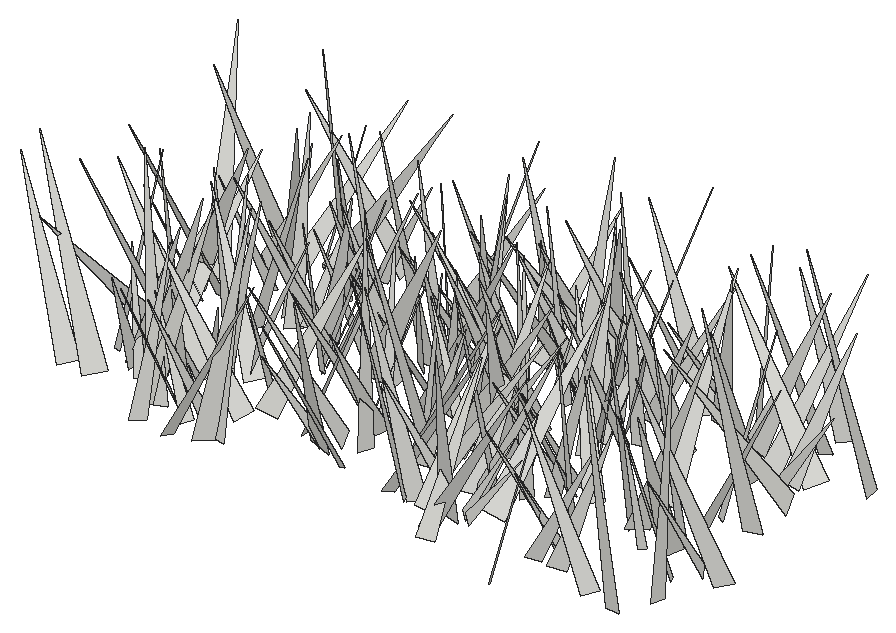
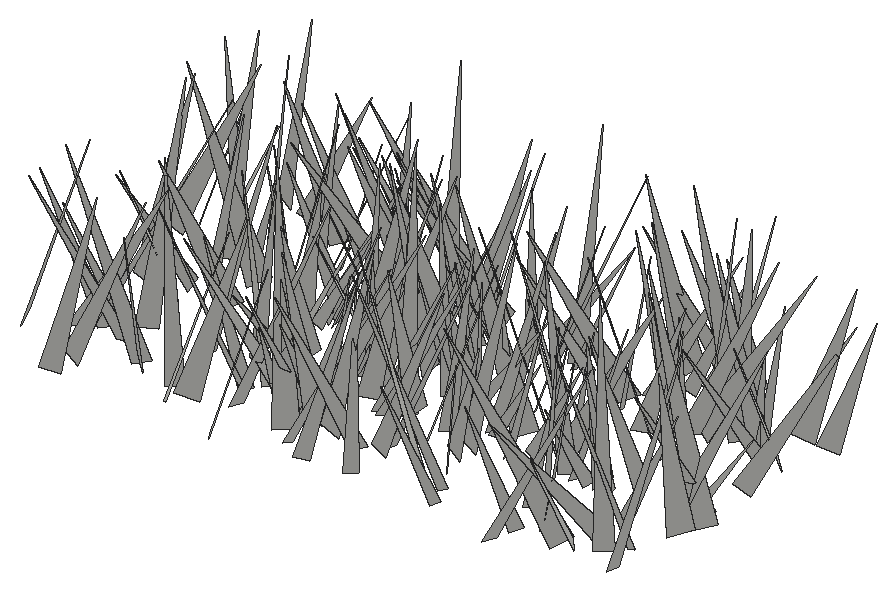
# SketchUp Ruby script. Lengths in inches.
U = 1.inch
M = Sketchup.active_model
def pt(a) = Geom::Point3d.new(a.map { |v| v * U })
def face(e, loops, mat)
  f = e.add_face(loops[0].map { |a| pt(a) })
  loops[1..].each { |l| e.add_face(l.map { |a| pt(a) }).erase! }
  f.material = f.back_material = mat if mat
  f
end
# faces: each face lists its corners as indices into pts; further lists are holes
def faces(e, pts, list, mat = nil) = list.each { |f| face(e, (f[0].is_a?(Array) ? f : [f]).map { |l| l.map { |i| pts[i] } }, mat) }
# xy, xz, yz: faces in a plane at the given z, y or x. An outline is a flat list of corners, or four numbers for a rectangle; further outlines are holes
def ring(l) = l.size == 4 ? [[l[0], l[1]], [l[2], l[1]], [l[2], l[3]], [l[0], l[3]]] : l.each_slice(2).to_a
def flat(e, list, mat, &to3) = list.each { |f| face(e, (f[0].is_a?(Array) ? f : [f]).map { |l| ring(l).map { |u, v| to3.(u, v) } }, mat) }
def xy(e, z, list, mat = nil) = flat(e, list, mat) { |x, y| [x, y, z] }
def xz(e, y, list, mat = nil) = flat(e, list, mat) { |x, z| [x, y, z] }
def yz(e, x, list, mat = nil) = flat(e, list, mat) { |y, z| [x, y, z] }
def lines(e, pts, list) = list.each { |a, b| e.add_line(pt(pts[a]), pt(pts[b])) }
# prism: a flat outline (further loops are holes) pulled along v
def prism(e, loops, v, mat = nil)
  f = face(e, loops, mat); d = Geom::Vector3d.new(v.map { |x| x * U })
  f.pushpull(f.normal.samedirection?(d) ? d.length : -d.length)
end
def box(e, o, s, mat = nil) = prism(e, [[o, [o[0] + s[0], o[1], o[2]], [o[0] + s[0], o[1] + s[1], o[2]], [o[0], o[1] + s[1], o[2]]]], [0, 0, s[2]], mat)
def at(x, y, z, deg = 0) = Geom::Transformation.translation(pt([x, y, z])) * Geom::Transformation.rotation(ORIGIN, Z_AXIS, deg.degrees)
def axes(o, x, y, z) = Geom::Transformation.new([*x, 0, *y, 0, *z, 0, *pt(o).to_a, 1])
def part(name) = M.definitions.add(name)
# library, detail: a bought-in or finely detailed component or shape, given as its bounding box
def library(name, o, s) = part(name).tap { |d| box(d.entities, o, s) }
def detail(e, o, s) = box(e.add_group.entities, o, s)
def put(e, d, t, mat = nil) = e.add_instance(d, t).tap { |i| i.material = mat if mat }
def group(e, t, mat = nil) = e.add_group.tap { |g| g.transformation = t; g.material = mat if mat }.entities
root = M.entities
c1 = part("fur_instance\#9")
p = [[0.8125,0,1.79],[0.67,-0.02,1.48],[0,-0.11,0],[0,0.11,0]]
faces(c1.entities,p,[[0,1,2,3]])
put(root,c1,axes([500.28,287.19,-21.66],[1.97558,6.78512,3.04566],[6.89111,-2.85534,1.89119],[-2.79761,-2.24188,6.80913]))
put(root,c1,axes([492.22,285.11,-21.66],[4.15865,3.49208,0.81847],[2.77358,-3.92559,2.6563],[-2.27416,1.59814,4.73636]))
put(root,c1,axes([462.6,291.13,-21.66],[-3.43989,-5.36661,0.1848],[-4.97328,3.26677,2.29397],[2.02515,-1.09328,5.94736]))
put(root,c1,axes([485.08,290.03,-21.66],[-0.53699,-7.34105,1.16615],[-7.27133,0.76139,1.44476],[1.5423,1.0337,7.21748]))
put(root,c1,axes([497.86,288,-21.66],[-2.44299,5.49091,1.30941],[5.27932,1.71736,2.64808],[-1.99837,-2.17564,5.395]))
put(root,c1,axes([465.14,287.3125,-21.66],[5.97099,-0.01983,0.33196],[-0.11666,-5.7151,1.75709],[-0.31141,1.76085,5.70664]))
put(root,c1,axes([492.93,291.41,-21.66],[-4.66281,-2.88259,0.04543],[-2.761,4.48988,1.50703],[0.82963,-1.25893,5.27068]))
put(root,c1,axes([473.41,291.95,-21.66],[-0.94018,-7.50089,0.47804],[-7.29693,1.02641,1.75419],[1.80188,0.24278,7.35324]))
put(root,c1,axes([484.875,288.33,-21.66],[6.3813,-2.25892,0.20905],[-2.20352,-6.02357,2.17449],[0.53935,2.11689,6.41056]))
put(root,c1,axes([492.47,289.16,-21.66],[3.58397,-3.64133,0.7361],[-3.60405,-3.15993,1.91614],[0.90107,1.84433,4.7363]))
put(root,c1,axes([465.87,290.28,-21.66],[0.12283,-4.44104,1.09952],[-4.1986,-0.54638,-1.73783],[-1.81756,0.96203,4.08875]))
put(root,c1,axes([462.5,287.67,-21.66],[4.91626,-1.03874,2.91243],[-2.03601,-5.20453,1.58061],[-2.3272,2.35896,4.76972]))
put(root,c1,axes([492.23,291.64,-21.66],[-3.17214,-2.54983,0.51656],[-2.07776,2.97317,1.9168],[1.56569,-1.22048,3.59026]))
put(root,c1,axes([494.35,289.11,-21.66],[3.63193,-4.05591,1.60644],[-4.34601,-3.18259,1.79036],[0.37856,2.37544,5.14159]))
put(root,c1,axes([485.71,286.98,-21.66],[-4.47907,3.89554,0.463],[3.44419,4.24137,-2.36643],[1.87807,1.51235,5.44401]))
put(root,c1,axes([467.35,288.15,-21.66],[-6.57541,3.25527,2.97746],[2.73361,7.20101,-1.83599],[3.46258,0.49673,7.10365]))
put(root,c1,axes([486.16,290.57,-21.66],[2.45066,3.05169,0.44917],[2.65928,-1.79957,-2.28257],[1.56295,-1.7231,3.17938]))
put(root,c1,axes([465.07,289.35,-21.66],[-1.27036,4.00789,0.19304],[3.62684,1.0603,1.85365],[-1.71652,-0.72583,3.77372]))
put(root,c1,axes([476.07,290.8125,-21.66],[-2.89235,-4.23355,0.19447],[-3.82387,2.50545,-2.32964],[-1.82723,1.45817,4.56743]))
put(root,c1,axes([482.33,290.4,-21.66],[0.18988,-6.4583,3.19895],[-6.79344,-1.22898,-2.07794],[-2.40669,2.95955,6.11783]))
put(root,c1,axes([473.21,292.5,-21.66],[-4.08154,-1.42978,0.42723],[-1.12455,3.76494,1.85644],[0.98091,-1.633,3.906]))
put(root,c1,axes([481.54,290.31,-21.66],[-6.3033,-3.29184,1.05702],[-3.45211,6.11366,-1.54635],[0.19083,1.86335,6.94094]))
put(root,c1,axes([474.08,293.63,-21.66],[-6.53247,-2.60599,0.49941],[-2.30056,6.22381,2.3844],[1.32211,-2.04617,6.61657]))
put(root,c1,axes([468.03,288.6875,-21.66],[2.36714,6.37429,1.14743],[6.22522,-2.57637,1.46983],[-1.78738,-0.5313,6.63886]))
put(root,c1,axes([485.68,290.84,-21.66],[2.51119,2.94201,0.30611],[2.79372,-2.22715,-1.51331],[0.97173,-1.19981,3.55969]))
put(root,c1,axes([482.82,292.76,-21.66],[-4.59731,-1.23154,0.33008],[-1.08177,4.4213,1.42926],[0.67485,-1.30242,4.53973]))
put(root,c1,axes([458.12,292.93,-21.66],[4.10212,-1.60455,0.85508],[-1.23063,-4.00368,-1.60913],[-1.3384,-1.23658,4.10033]))
put(root,c1,axes([467.38,292.04,-21.66],[-6.03456,2.61232,0.13904],[2.52964,5.73798,1.98392],[-0.66667,-1.87372,6.2693]))
put(root,c1,axes([461.77,289.54,-21.66],[6.32729,-2.1008,2.73388],[-3.01636,-6.1404,2.26257],[-1.67006,3.13117,6.27127]))
put(root,c1,axes([501.77,289.8,-21.66],[-7.13651,-0.0123,2.39844],[-0.61978,7.28244,-1.80677],[2.31701,1.91008,6.90402]))
put(root,c1,axes([462.29,289.82,-21.66],[0.0482,8.00911,1.76337],[7.92916,-0.49572,2.03478],[-2.09374,-1.69294,7.74648]))
put(root,c1,axes([454.68,290.63,-21.66],[-3.24359,5.98487,0.42852],[5.75195,2.96279,2.1587],[-1.708,-1.38792,6.45597]))
put(root,c1,axes([456.8,290.5625,-21.66],[-3.17251,7.14398,0.8627],[6.87917,2.73438,2.65436],[-2.11131,-1.82544,7.35225]))
put(root,c1,axes([459.48,293.04,-21.66],[3.88235,-7.18309,1.19208],[-7.15051,-3.50623,2.16032],[1.37403,2.04942,7.87416]))
put(root,c1,axes([494.06,291.3125,-21.66],[-3.8782,-4.63911,2.52217],[-5.26639,3.62608,-1.42825],[0.38461,2.87286,5.87554]))
put(root,c1,axes([501.56,294.53,-21.66],[-3.93384,-2.91751,0.42121],[-2.51987,3.69278,2.04402],[1.52955,-1.41982,4.45073]))
put(root,c1,axes([498.68,295.03,-21.66],[5.9537,-4.05045,0.58701],[-3.75603,-5.81897,-2.05648],[-1.62572,-1.38951,6.90098]))
put(root,c1,axes([463.2,291.48,-21.66],[-7.60319,-2.30719,2.08818],[-2.71089,7.61771,-1.45385],[1.52798,2.03457,7.8114]))
put(root,c1,axes([483.4,289.82,-21.66],[-1.05391,6.67902,0.37292],[6.52998,1.10912,-1.41007],[1.4518,-0.14015,6.613]))
put(root,c1,axes([458.13,293.06,-21.66],[3.9818,-4.86666,0.84742],[-4.90357,-3.76221,1.43455],[0.59785,1.55519,6.12218]))
put(root,c1,axes([500.71,292.46,-21.66],[-4.67684,-2.75,0.36196],[-2.71074,4.38122,-1.73872],[-0.58771,1.67594,5.13928]))
put(root,c1,axes([475.25,295.77,-21.66],[4.02503,-3.95124,0.17731],[-3.62061,-3.78264,-2.10414],[-1.59215,-1.38705,5.23314]))
put(root,c1,axes([480.17,290.26,-21.66],[6.45135,0.1489,0.38361],[-0.04006,-5.77049,2.9136],[-0.40954,2.91007,5.75787]))
put(root,c1,axes([484.93,293.11,-21.66],[5.1253,5.35023,0.94765],[5.22805,-4.50107,-2.86349],[1.48003,-2.62814,6.83331]))
put(root,c1,axes([467.77,294.59,-21.66],[-3.99319,-2.60087,1.40659],[-2.16034,4.18012,1.59628],[2.0189,-0.6713,4.49021]))
put(root,c1,axes([459.36,291.79,-21.66],[-0.27528,4.26527,0.41219],[4.05575,0.12601,1.40472],[-1.38323,-0.47937,4.03672]))
put(root,c1,axes([462.17,293.75,-21.66],[-3.051,-7.21191,1.32168],[-6.61753,2.09219,-3.8598],[-3.15701,2.58422,6.81338]))
put(root,c1,axes([503.68,293.95,-21.66],[-2.36054,6.29762,2.85628],[6.53149,1.03928,3.10644],[-2.27111,-3.55673,5.96508]))
put(root,c1,axes([479.49,292.14,-21.66],[7.04502,0.38941,0.11832],[0.34745,-6.82295,1.76766],[-0.21195,1.75889,6.83077]))
put(root,c1,axes([462.61,294.39,-21.66],[-6.95314,3.37085,0.59923],[3.40426,6.66259,2.02209],[-0.36434,-2.07731,7.45788]))
put(root,c1,axes([479.64,294.11,-21.66],[3.48254,-4.50934,1.30252],[-4.66936,-3.1635,1.53235],[0.47726,1.95368,5.48763]))
put(root,c1,axes([462.06,295.52,-21.66],[-0.71595,-3.844,0.50308],[-3.36107,0.87042,1.86752],[1.93201,0.08975,3.4353]))
put(root,c1,axes([485.99,293.68,-21.66],[-6.23091,-2.8217,1.23434],[-3.03851,6.08694,-1.42355],[0.50305,1.81577,6.69027]))
put(root,c1,axes([455.6875,297.9,-21.66],[3.04305,-5.48081,0.27728],[-4.42438,-2.6378,-3.58374],[-3.24669,-1.54241,5.14356]))
put(root,c1,axes([481.29,294.26,-21.66],[4.41498,5.25807,0.18984],[4.81628,-3.93899,-2.90917],[2.11822,-2.00311,6.21901]))
put(root,c1,axes([479.53,295.18,-21.66],[-2.64388,-6.79077,2.11498],[-6.99476,2.07362,-2.08599],[-1.28885,2.67645,6.98236]))
put(root,c1,axes([471.73,298.14,-21.66],[-4.9139,-3.74374,0.55427],[-3.15126,4.55055,2.79845],[2.0958,-1.9355,5.50733]))
put(root,c1,axes([494.1875,296.66,-21.66],[-6.11732,-3.75265,2.76683],[-3.28898,6.70851,1.82699],[3.3046,-0.26993,6.94018]))
put(root,c1,axes([475.89,293.37,-21.66],[-7.47088,0.3057,1.86762],[-0.12287,7.51123,-1.721],[1.88848,1.69808,7.27638]))
put(root,c1,axes([463.24,295.18,-21.66],[2.35807,6.09522,2.44102],[6.53945,-1.94795,-1.45322],[0.58808,-2.77931,6.37184]))
put(root,c1,axes([471.66,292.61,-21.66],[5.28462,2.45266,0.54887],[2.09175,-5.00051,2.20534],[-1.39334,1.79538,5.39252]))
put(root,c1,axes([496.86,294.43,-21.66],[0.33091,4.05955,1.18914],[3.81261,-0.80293,1.68011],[-1.83248,-0.93747,3.71034]))
put(root,c1,axes([483.33,297.95,-21.66],[6.57894,-4.30915,0.69378],[-4.10201,-6.53322,-1.6802],[-1.49116,-1.03963,7.68298]))
put(root,c1,axes([488.18,297.48,-21.66],[-4.30266,-2.43803,0.04686],[-2.30354,4.09498,1.544],[0.79994,-1.32144,4.69819]))
put(root,c1,axes([468.21,293.21,-21.66],[-2.47927,6.31853,1.78834],[5.49074,3.04318,-3.14001],[3.60191,-0.28983,6.01756]))
put(root,c1,axes([487.06,291.96,-21.66],[-2.37553,7.32496,0.20013],[6.77476,2.27563,-2.87444],[2.79244,0.71043,7.14393]))
put(root,c1,axes([489.23,297.04,-21.66],[-2.79932,-5.24784,0.26282],[-5.09915,2.64134,-1.57068],[-1.26789,0.96362,5.73663]))
put(root,c1,axes([479.86,296.21,-21.66],[5.30447,3.34271,0.68413],[3.37643,-4.96043,-1.94241],[0.49141,-1.99988,5.96139]))
put(root,c1,axes([479.98,296.75,-21.66],[3.5795,-7.50714,1.0436],[-6.77337,-2.6505,4.166],[3.40115,2.62237,7.19823]))
put(root,c1,axes([484.29,293.2,-21.66],[-4.73234,6.09922,1.47861],[5.53404,4.92888,-2.61961],[2.95993,0.53615,7.26177]))
put(root,c1,axes([464.15,296.26,-21.66],[4.41432,4.17138,0.78555],[4.1779,-4.06951,-1.86761],[0.75011,-1.88212,5.77916]))
put(root,c1,axes([495.09,296.125,-21.66],[6.69732,-3.52244,1.21858],[-3.71872,-6.48437,1.69431],[-0.25228,2.07171,7.37503]))
put(root,c1,axes([456.86,294.37,-21.66],[-1.28039,5.01222,0.36244],[4.5705,1.31696,-2.06622],[2.08908,0.19072,4.74262]))
put(root,c1,axes([456.03,293.74,-21.66],[3.80784,5.11048,0.67094],[4.57882,-3.73693,2.47721],[-2.36675,0.99257,5.87197]))
put(root,c1,axes([463.74,294.83,-21.66],[1.51119,6.34193,0.92742],[6.21067,-1.68435,1.39797],[-1.58356,-0.55387,6.36784]))
put(root,c1,axes([489,298.05,-21.66],[-0.33006,-3.76044,0.39687],[-3.50265,0.15395,-1.45434],[-1.42474,0.49269,3.4835]))
put(root,c1,axes([465.05,296.04,-21.66],[-4.13597,4.87198,0.25098],[4.78591,3.98836,1.44689],[-0.94567,-1.12348,6.22487]))
put(root,c1,axes([487.36,294.91,-21.66],[-7.91635,-0.39433,1.24518],[-0.80795,7.48837,-2.76517],[1.02625,2.85367,7.42819]))
put(root,c1,axes([498.09,296.79,-21.66],[1.91991,5.69676,2.84026],[5.7974,-2.78995,1.67703],[-2.62873,-1.9923,5.77292]))
put(root,c1,axes([478.6,295.625,-21.66],[2.37609,4.94692,0.8109],[4.47755,-2.49789,2.11838],[-2.25414,0.25283,5.06264]))
put(root,c1,axes([480.75,297.25,-21.66],[-2.13288,4.47426,0.69403],[4.36785,1.83113,1.61826],[-1.19274,-1.2953,4.68502]))
put(root,c1,axes([483.03,301.42,-21.66],[6.13444,-4.45258,1.42838],[-3.84619,-6.14459,-2.6359],[-2.65943,-1.38408,7.10696]))
put(root,c1,axes([462.23,297.14,-21.66],[-5.98582,-0.44068,0.88109],[-0.67667,5.78235,-1.70504],[0.71598,1.78068,5.75475]))
put(root,c1,axes([488.52,296.04,-21.66],[6.48387,0.57283,2.72889],[-0.5216,-6.53637,2.61139],[-2.73914,2.60063,5.96233]))
put(root,c1,axes([483.16,300.95,-21.66],[-6.61379,-2.13915,0.88077],[-1.88588,6.53057,1.69974],[1.33985,-1.36736,6.74011]))
put(root,c1,axes([477.05,300.01,-21.66],[-0.17668,-5.97479,1.5156],[-5.97573,0.53792,1.42395],[1.51188,1.4279,5.80532]))
put(root,c1,axes([473.65,296.73,-21.66],[3.6245,2.89722,0.22495],[2.66528,-3.45765,1.58821],[-1.15791,1.11007,4.35987]))
put(root,c1,axes([481.72,301.33,-21.66],[0.79588,-7.21699,0.96951],[-7.03929,-1.01213,-1.75565],[-1.86367,0.74092,7.04528]))
put(root,c1,axes([475.84,299.15,-21.66],[7.56022,-3.29271,0.03526],[-3.23696,-7.41517,1.59297],[0.60437,1.47429,8.09082]))
put(root,c1,axes([490.92,297.02,-21.66],[-1.83761,6.5724,0.07775],[6.30696,1.74042,1.94227],[-1.85059,-0.59481,6.54223]))
put(root,c1,axes([480.63,299.64,-21.66],[4.14208,3.82367,0.06036],[3.46383,-3.71363,-2.44781],[1.62049,-1.8356,5.07794]))
put(root,c1,axes([470.43,300.75,-21.66],[3.82613,-7.13137,0.63835],[-6.75778,-3.35774,2.99351],[2.36564,1.94225,7.51895]))
put(root,c1,axes([500.92,300.21,-21.66],[-1.04276,-7.37455,2.60053],[-7.71345,0.53914,-1.56404],[-1.28435,2.74945,7.28184]))
put(root,c1,axes([467.01,301.19,-21.66],[-0.65869,-6.64833,1.3688],[-6.16249,0.00919,-2.92087],[-2.84565,1.51902,6.00855]))
put(root,c1,axes([467.14,300.78,-21.66],[4.68379,1.41709,0.13919],[1.37897,-4.39495,-1.65779],[0.35492,-1.62533,4.60411]))
put(root,c1,axes([488.79,303.03,-21.66],[-6.12859,-4.53414,1.24355],[-3.97845,6.08997,2.59781],[2.50535,-1.42065,7.16724]))
put(root,c1,axes([488.38,300.61,-21.66],[5.36268,3.16176,1.79895],[3.56295,-5.21159,-1.4615],[-0.73371,-2.1986,6.05138]))
put(root,c1,axes([474.11,297.625,-21.66],[0.39127,5.5531,0.09038],[5.24022,-0.39914,1.8382],[-1.83989,0.04412,5.25462]))
put(root,c1,axes([479.92,298.2,-21.66],[-7.4216,0.05563,3.73189],[-0.80703,8.0859,-1.72548],[3.64401,1.90407,7.21845]))
put(root,c1,axes([472.16,301.65,-21.66],[-6.75805,0.02177,1.99006],[0.56326,6.77748,1.83863],[1.90881,-1.92284,6.50317]))
put(root,c1,axes([467.12,300.11,-21.66],[6.01088,3.96881,0.98389],[4.08835,-5.80352,-1.56674],[0.06989,-1.84874,7.03046]))
put(root,c1,axes([467.625,299.45,-21.66],[1.94279,3.86541,2.10519],[3.74501,-2.66073,1.42935],[-2.3126,-1.06149,4.08323]))
put(root,c1,axes([485.15,297.89,-21.66],[3.44077,4.42208,0.21812],[4.18127,-3.33634,1.68138],[-1.45578,0.8691,5.34478]))
put(root,c1,axes([474.41,301.45,-21.66],[-2.08934,-4.39389,0.06996],[-3.98317,1.86084,-2.08523],[-1.85622,0.95264,4.39584]))
put(root,c1,axes([483.43,299.07,-21.66],[-4.4668,1.24969,0.75909],[0.98308,4.37301,-1.41442],[1.08236,1.18546,4.4174]))
put(root,c1,axes([500.48,304.37,-21.66],[-7.29463,-2.71144,0.02018],[-2.47986,6.69465,3.09773],[1.09665,-2.89718,7.13916]))
put(root,c1,axes([498.13,298.85,-21.66],[5.03908,0.51167,0.65236],[0.18588,-4.61324,2.18248],[-0.80798,2.12978,4.57066]))
put(root,c1,axes([454.51,302.97,-21.66],[3.10816,-7.62871,0.22312],[-7.12075,-2.81203,3.04879],[2.74626,1.34273,7.65263]))
put(root,c1,axes([488.52,300.85,-21.66],[-3.99392,-3.16377,0.39905],[-3.06383,3.62986,-1.88605],[-0.88412,1.71311,4.73326]))
put(root,c1,axes([474.39,303.47,-21.66],[5.34642,-2.10558,1.0321],[-1.67954,-5.23165,-1.97278],[-1.63641,-1.50973,5.39684]))
put(root,c1,axes([480.85,303.2,-21.66],[4.14575,-5.15062,1.64406],[-4.88287,-4.45639,-1.64839],[-2.32151,0.17524,6.40304]))
put(root,c1,axes([477.65,303.45,-21.66],[7.83218,-2.47016,1.5817],[-2.12062,-7.88445,-1.81244],[-2.02643,-1.29626,8.00998]))
put(root,c1,axes([486.71,302.35,-21.66],[6.48852,0.93317,0.66882],[1.0636,-6.33108,-1.48501],[-0.43231,-1.57025,6.38486]))
put(root,c1,axes([464.62,303.35,-21.66],[-4.80536,-1.45342,1.08645],[-0.98448,4.67157,1.89512],[1.52434,-1.5647,4.64891]))
put(root,c1,axes([456.87,303.02,-21.66],[-2.83632,-6.0499,0.28173],[-5.90232,2.69141,-1.62612],[-1.35766,0.93829,6.48088]))
put(root,c1,axes([467.35,301.57,-21.66],[5.84897,4.9177,0.90335],[4.92852,-5.43629,-2.31659],[0.84231,-2.33947,7.282]))
put(root,c1,axes([465.28,303.01,-21.66],[0.87943,-6.58228,1.27772],[-6.45662,-0.48373,1.95201],[1.80858,1.47376,6.34739]))
put(root,c1,axes([496.97,304.83,-21.66],[6.98894,-3.62557,1.01436],[-3.15649,-6.80873,-2.58782],[-2.05189,-1.87497,7.43594]))
put(root,c1,axes([479.375,304.2,-21.66],[-5.28354,-0.86585,0.73138],[-0.45173,4.80676,2.42722],[1.0395,-2.31209,4.77222]))
put(root,c1,axes([456.21,301.82,-21.66],[-2.80536,-2.90649,0.0794],[-2.63209,2.49174,-1.78533],[-1.23535,1.29136,3.62358]))
put(root,c1,axes([471.7,302.2,-21.66],[-2.56697,2.61634,0.35758],[2.51502,2.27032,1.44317],[-0.80484,-1.25014,3.36925]))
put(root,c1,axes([482.8125,300.3125,-21.66],[0.07199,5.81915,0.58708],[5.58747,-0.24194,1.7129],[-1.72841,-0.53974,5.5618]))
put(root,c1,axes([472,303.68,-21.66],[-2.28168,-4.43341,1.38047],[-4.1851,2.6298,1.52839],[2.0114,0.44265,4.74608]))
put(root,c1,axes([492.07,304.9,-21.66],[-7.41474,-1.37074,2.09218],[-0.74138,7.45582,2.25736],[2.38883,-1.94072,7.19456]))
put(root,c1,axes([468.4375,302.72,-21.66],[-1.09532,-3.977,1.33167],[-3.82769,0.38536,-1.99748],[-1.71426,1.68065,3.6092]))
put(root,c1,axes([461.02,301.15,-21.66],[5.70541,0.17051,1.69377],[-0.31532,-5.71566,1.63753],[-1.67287,1.65887,5.46803]))
put(root,c1,axes([498.32,300.28,-21.66],[3.77258,4.9169,0.38845],[4.64704,-3.70729,1.79444],[-1.65279,0.7995,5.93196]))
put(root,c1,axes([494.63,299.52,-21.66],[-5.35866,5.61511,0.59327],[5.12673,5.1813,-2.73266],[2.36603,1.4904,7.2648]))
put(root,c1,axes([474.01,306.36,-21.66],[-4.88167,-3.98465,0.29136],[-3.56929,4.55624,2.50876],[1.79514,-1.77658,5.7805]))
put(root,c1,axes([478.73,304.23,-21.66],[-5.72955,1.74546,0.28048],[1.75274,5.48455,1.67353],[-0.23061,-1.68113,5.75097]))
put(root,c1,axes([455.63,301.26,-21.66],[-0.63862,5.35473,0.03552],[5.1577,0.62471,-1.44573],[1.43964,0.13724,5.19527]))
put(root,c1,axes([486.59,305.99,-21.66],[6.70588,0.95076,0.50826],[1.07552,-6.12086,-2.74035],[-0.07444,-2.78609,6.19381]))
put(root,c1,axes([472.22,304.12,-21.66],[1.71463,6.79892,3.94816],[7.36353,-2.80488,1.63226],[-2.7553,-3.26505,6.81916]))
put(root,c1,axes([469.95,302.88,-21.66],[-7.13799,-1.18277,0.6594],[-1.323,6.84565,-2.04241],[0.28881,2.12669,6.94107]))
put(root,c1,axes([486.875,301.35,-21.66],[-6.53703,2.92768,0.70077],[2.53956,6.26275,-2.47462],[1.61648,2.00045,6.72163]))
put(root,c1,axes([475.85,307.09,-21.66],[-6.75502,-2.37628,0.59319],[-2.11002,6.52988,2.13012],[1.24354,-1.82836,6.83664]))
put(root,c1,axes([481.92,307.35,-21.66],[-0.45254,-7.13046,0.09555],[-6.72101,0.39447,-2.39372],[-2.38342,0.24148,6.7319]))
put(root,c1,axes([458.82,305.49,-21.66],[-0.44719,-4.16584,0.88919],[-4.01944,0.11666,-1.47491],[-1.41032,0.98845,3.92158]))
put(root,c1,axes([462.83,302.63,-21.66],[-6.34351,2.24327,1.15963],[1.89857,6.30395,-1.80908],[1.66506,1.35834,6.48071]))
put(root,c1,axes([482.71,307.1,-21.66],[-6.34287,-0.8603,1.40577],[-0.30586,6.10717,2.3574],[1.61949,-2.21602,5.95103]))
put(root,c1,axes([463.48,303.14,-21.66],[-2.96386,2.60362,0.59977],[2.15648,2.85999,-1.75873],[1.5774,0.98217,3.53132]))
put(root,c1,axes([461.72,303.46,-21.66],[4.93577,0.48548,2.66433],[-0.37318,-5.36398,1.66873],[-2.68236,1.63958,4.67042]))
put(root,c1,axes([498.68,305.21,-21.66],[1.93678,-3.59499,0.72466],[-3.24209,-1.29543,2.2385],[1.71404,1.61186,3.41529]))
put(root,c1,axes([477.37,302.76,-21.66],[-6.45449,2.84921,1.13675],[2.42101,6.35763,-2.18855],[1.88385,1.59157,6.70736]))
put(root,c1,axes([464.63,307.71,-21.66],[4.72297,-1.05883,1.70864],[-0.28791,-4.67444,-2.10088],[-1.98939,-1.83725,4.36049]))
put(root,c1,axes([488.65,304.38,-21.66],[1.70019,7.5386,2.42367],[7.33263,-2.43467,2.42902],[-2.9895,-1.68439,7.33628]))
put(root,c1,axes([486.35,303.23,-21.66],[-3.43381,3.18637,0.41007],[2.54254,3.06224,-2.50406],[1.96382,1.60682,3.959]))
put(root,c1,axes([457.54,309.1,-21.66],[7.63705,-2.12328,0.08153],[-2.0044,-7.29978,-2.35267],[-0.70524,-2.24596,7.56953]))
put(root,c1,axes([487.33,307.1,-21.66],[1.64693,-4.65446,0.85777],[-4.4282,-1.19483,2.01879],[1.67056,1.42146,4.50564]))
put(root,c1,axes([482.33,309.43,-21.66],[2.66865,-7.95792,0.14871],[-7.80747,-2.5868,1.68053],[1.54726,0.67254,8.22351]))
put(root,c1,axes([482.03,305.48,-21.66],[-6.19983,-0.76734,1.02255],[-1.02443,6.01091,-1.70052],[0.76483,1.83095,6.01123]))
put(root,c1,axes([486.62,308.9375,-21.66],[-7.42366,-0.80204,0.92134],[-0.52005,7.2098,2.08597],[1.1053,-1.9946,7.16957]))
put(root,c1,axes([462.09,309.41,-21.66],[5.97611,0.87511,2.00016],[1.66713,-5.59279,-2.53411],[-1.40966,-2.90435,5.48252]))
put(root,c1,axes([472.375,305.38,-21.66],[0.67019,6.07953,1.22269],[5.42193,-1.17133,2.85227],[-3.0097,-0.75637,5.41058]))
put(root,c1,axes([476.1875,308,-21.66],[-1.63613,-6.00923,1.56488],[-6.02721,1.14742,-1.89548],[-1.49415,1.95172,5.93253]))
put(root,c1,axes([455.2,304.5,-21.66],[-6.50457,4.89284,0.5628],[4.72218,6.46057,-1.59001],[1.39918,0.94188,7.98255]))
put(root,c1,axes([498.96,306.3,-21.66],[-0.64371,5.67181,1.6895],[5.48083,1.21245,-1.9821],[2.23257,-1.34117,5.35305]))
put(root,c1,axes([491.06,309.48,-21.66],[0.69431,-7.1025,1.01226],[-6.95299,-0.41552,1.85354],[1.7681,1.15502,6.89145]))
put(root,c1,axes([500.24,307.3,-21.66],[-5.51381,4.9525,0.02994],[4.6746,5.18943,2.47955],[-1.63592,-1.86355,6.98435]))
put(root,c1,axes([481.2,310.63,-21.66],[-6.30471,-1.37126,0.42808],[-1.05468,5.72683,2.8114],[0.97532,-2.67133,5.80738]))
put(root,c1,axes([456.37,307.89,-21.66],[3.98085,5.13777,1.04709],[4.9615,-3.26572,-2.83883],[1.69606,-2.50573,5.84679]))
put(root,c1,axes([485.77,306.03,-21.66],[-3.80527,0.70423,0.62745],[0.3357,3.44844,-1.83447],[0.88144,1.72686,3.40746]))
put(root,c1,axes([487.24,307.43,-21.66],[3.70489,5.29932,0.63458],[5.07029,-3.25343,-2.43293],[1.66665,-1.88258,5.99082]))
put(root,c1,axes([484.94,305.61,-21.66],[-5.93651,2.05948,0.4431],[1.83167,5.70073,-1.95618],[1.04056,1.71471,5.97135]))
put(root,c1,axes([490.35,311.35,-21.66],[-3.99829,-3.957,0.07334],[-3.50173,3.58563,2.55553],[1.84422,-1.77059,5.01133]))
put(root,c1,axes([480.05,307.96,-21.66],[-1.59145,-6.67923,2.98055],[-7.18236,0.85085,-1.92829],[-1.38185,3.26993,6.58988]))
put(root,c1,axes([471.7,306.85,-21.66],[-4.19914,-2.372,1.71601],[-2.90919,3.71707,-1.98087],[0.32817,2.60017,4.39719]))
put(root,c1,axes([455.65,310.61,-21.66],[-7.05336,-2.15617,1.71578],[-1.62887,7.06566,2.18314],[2.22256,-1.66441,7.04506]))
put(root,c1,axes([494.52,308.39,-21.66],[2.05152,-6.6713,2.37008],[-6.64568,-0.96384,3.03943],[2.44098,2.98279,6.28306]))
put(root,c1,axes([482.3,307.13,-21.66],[0.05703,4.78722,0.58826],[4.57544,0.13244,-1.52137],[1.52606,-0.57598,4.5394]))
put(root,c1,axes([482.55,306.09,-21.66],[-4.05374,2.9207,0.15477],[2.65047,3.78022,-1.91631],[1.23673,1.47198,4.61422]))
put(root,c1,axes([479.28,311.72,-21.66],[5.03177,-2.92165,1.14225],[-2.20313,-4.82824,-2.64459],[-2.23316,-1.81978,5.18275]))
put(root,c1,axes([503.62,308.5,-21.66],[-7.70081,-2.50661,0.76749],[-2.60656,7.57519,-1.4131],[0.27927,1.58364,7.97425]))
put(root,c1,axes([475.85,311.18,-21.66],[5.48383,-1.63022,0.30334],[-1.45467,-5.23263,-1.82362],[-0.79597,-1.66854,5.42259]))
put(root,c1,axes([470.08,309.33,-21.66],[3.77376,6.10396,1.49671],[5.76595,-2.66802,-3.65722],[2.50047,-3.05991,6.17449]))
put(root,c1,axes([463.42,307.28,-21.66],[-7.24108,-2.76695,1.69952],[-3.23599,6.49389,-3.21487],[0.2698,3.62643,7.05364]))
put(root,c1,axes([496.91,306.99,-21.66],[1.06363,7.1406,0.14161],[6.98782,-1.01087,-1.51263],[1.47601,-0.35985,7.05914]))
put(root,c1,axes([485.63,305.75,-21.66],[6.81061,4.1437,0.72104],[3.52808,-6.3754,3.31382],[-2.28972,2.50169,7.25074]))
put(root,c1,axes([481.43,307.5,-21.66],[-6.63675,3.07759,1.929],[2.57186,6.8191,-2.03087],[2.56478,1.12578,7.02806]))
put(root,c1,axes([470.89,309.86,-21.66],[7.00496,3.81978,0.96353],[3.93839,-6.83549,-1.53416],[-0.09034,-1.80938,7.82984]))
put(root,c1,axes([489.6,310.11,-21.66],[-4.16416,5.80884,2.0419],[6.1268,3.66414,2.07088],[-0.6118,-2.84317,6.84063]))
put(root,c1,axes([477.32,308.5625,-21.66],[-0.99691,5.86129,1.26655],[5.41282,1.43213,-2.36709],[2.58075,-0.73958,5.45394]))
put(root,c1,axes([498.29,310.65,-21.66],[-2.5015,-6.23633,1.72664],[-6.18785,1.76379,-2.59425],[-1.89304,2.47545,6.19832]))
put(root,c1,axes([463.37,310.46,-21.66],[3.09859,-2.8989,0.71648],[-2.92503,-2.73871,1.56906],[0.60101,1.61681,3.94246]))
put(root,c1,axes([485.45,313.0625,-21.66],[-4.40501,-3.46188,0.56585],[-3.18391,4.32713,1.68747],[1.47225,-1.00011,5.34239]))
put(root,c1,axes([460.18,309.96,-21.66],[5.69226,-5.26322,0.96159],[-5.00885,-4.7486,3.65927],[1.88086,3.28288,6.8347]))
put(root,c1,axes([463.9,312.49,-21.66],[-7.08449,-0.21202,0.14595],[-0.16992,6.87165,1.73429],[0.19334,-1.72965,6.8722]))
put(root,c1,axes([494.42,308.67,-21.66],[3.23969,5.31398,1.47982],[4.81259,-3.56155,2.25346],[-2.69577,0.02794,5.80137]))
put(root,c1,axes([469.3,311.02,-21.66],[1.72384,-3.5656,0.8716],[-3.29525,-1.07913,2.10276],[1.61693,1.60212,3.35612]))
put(root,c1,axes([458.59,307.78,-21.66],[-3.50989,5.55769,0.51718],[4.45011,3.15505,-3.70364],[3.36927,1.62248,5.4305]))
put(root,c1,axes([498.33,312.7,-21.66],[-3.08305,4.83073,2.80211],[5.58378,2.72141,1.452],[0.09585,-3.15451,5.54372]))
put(root,c1,axes([459.51,309.68,-21.66],[3.36886,3.17868,0.5186],[2.75759,-3.23451,1.91201],[-1.66392,1.0752,4.2187]))
